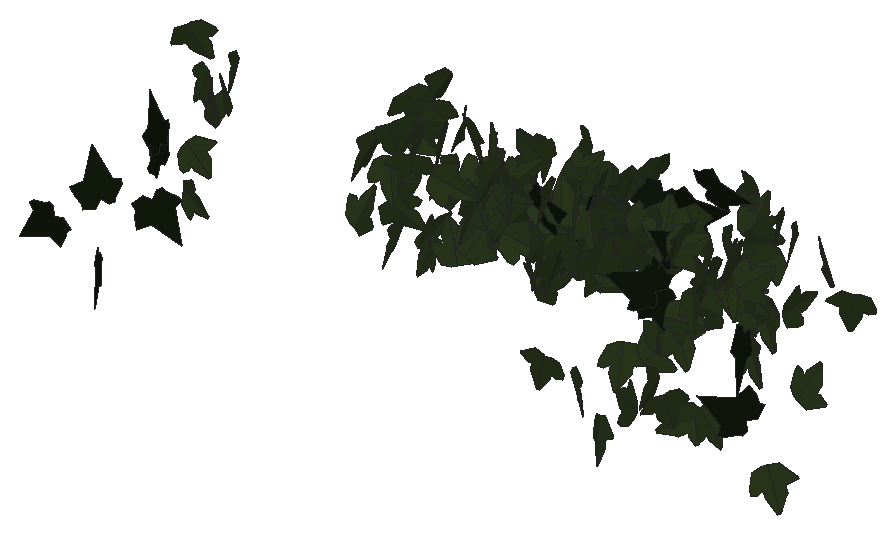
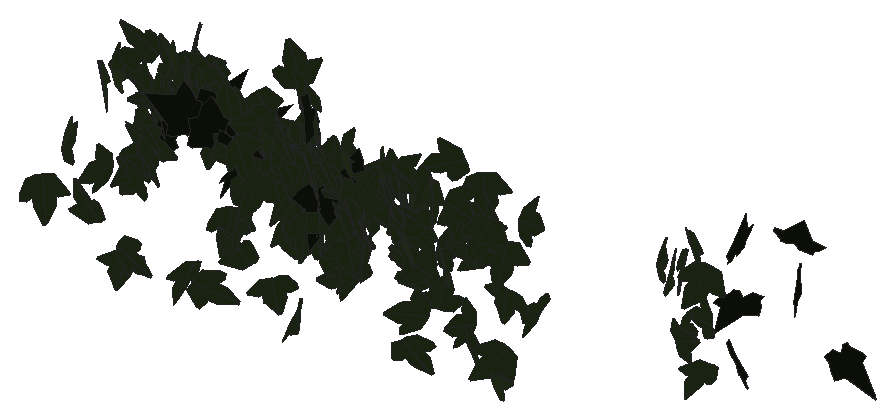
# SketchUp Ruby script. Lengths in inches.
U = 1.inch
M = Sketchup.active_model
def pt(a) = Geom::Point3d.new(a.map { |v| v * U })
def face(e, loops, mat)
  f = e.add_face(loops[0].map { |a| pt(a) })
  loops[1..].each { |l| e.add_face(l.map { |a| pt(a) }).erase! }
  f.material = f.back_material = mat if mat
  f
end
# faces: each face lists its corners as indices into pts; further lists are holes
def faces(e, pts, list, mat = nil) = list.each { |f| face(e, (f[0].is_a?(Array) ? f : [f]).map { |l| l.map { |i| pts[i] } }, mat) }
# xy, xz, yz: faces in a plane at the given z, y or x. An outline is a flat list of corners, or four numbers for a rectangle; further outlines are holes
def ring(l) = l.size == 4 ? [[l[0], l[1]], [l[2], l[1]], [l[2], l[3]], [l[0], l[3]]] : l.each_slice(2).to_a
def flat(e, list, mat, &to3) = list.each { |f| face(e, (f[0].is_a?(Array) ? f : [f]).map { |l| ring(l).map { |u, v| to3.(u, v) } }, mat) }
def xy(e, z, list, mat = nil) = flat(e, list, mat) { |x, y| [x, y, z] }
def xz(e, y, list, mat = nil) = flat(e, list, mat) { |x, z| [x, y, z] }
def yz(e, x, list, mat = nil) = flat(e, list, mat) { |y, z| [x, y, z] }
def lines(e, pts, list) = list.each { |a, b| e.add_line(pt(pts[a]), pt(pts[b])) }
# prism: a flat outline (further loops are holes) pulled along v
def prism(e, loops, v, mat = nil)
  f = face(e, loops, mat); d = Geom::Vector3d.new(v.map { |x| x * U })
  f.pushpull(f.normal.samedirection?(d) ? d.length : -d.length)
end
def box(e, o, s, mat = nil) = prism(e, [[o, [o[0] + s[0], o[1], o[2]], [o[0] + s[0], o[1] + s[1], o[2]], [o[0], o[1] + s[1], o[2]]]], [0, 0, s[2]], mat)
def at(x, y, z, deg = 0) = Geom::Transformation.translation(pt([x, y, z])) * Geom::Transformation.rotation(ORIGIN, Z_AXIS, deg.degrees)
def axes(o, x, y, z) = Geom::Transformation.new([*x, 0, *y, 0, *z, 0, *pt(o).to_a, 1])
def part(name) = M.definitions.add(name)
# library, detail: a bought-in or finely detailed component or shape, given as its bounding box
def library(name, o, s) = part(name).tap { |d| box(d.entities, o, s) }
def detail(e, o, s) = box(e.add_group.entities, o, s)
def put(e, d, t, mat = nil) = e.add_instance(d, t).tap { |i| i.material = mat if mat }
def group(e, t, mat = nil) = e.add_group.tap { |g| g.transformation = t; g.material = mat if mat }.entities
root = M.entities
M.materials.add("efeu1").color = [18, 25, 13]
M.materials.add("efeu2").color = [43, 57, 29]
c1 = part("ivyleaf_9")
p = [[1.54,2.16,1.25],[1.36,2.04,1.19],[-0.21,0.99,0.68],[-0.71,1.11,0.82],[-0.85,0.86,0.67],[-0.8,0.17,0.21],
  [-0.9,-0.01,0.1],[-0.67,-0.16,-0.02],[-0.08,-0.08,-0.05],[-0.03,-0.6,-0.4],[0.65,-0.88,-0.66],[0.83,-0.6,-0.49],
  [1.29,-0.42,-0.43],[1.8125,-0.07,-0.26],[1.21,0.44,0.15]]
faces(c1.entities,p,[[0,1,2,3,4,5,6,7,8,9,10,11,12,13,14]],"efeu1")
c2 = part("ivyleaf_10")
p = [[0,0.5,-0.03],[-0.0625,2.02,-0.43],[-0.19,2.01,-0.46],[-0.54,1.05,-0.29],[-0.52,0.625,-0.18],[-0.83,0.76,-0.28],
  [-1.16,0.64,-0.33],[-1.15,0.33,-0.24],[-0.77,-0.39,0.02],[-0.3,-0.51,0.16],[0.04,-0.48,0.23],[-0.02,2.01,-0.4375],
  [-0.06,2.01,-0.43],[0.04,-0.49,0.23],[0.67,-0.49,0.14],[1.38,0.36,-0.2],[1.375,0.51,-0.24],[0.81,0.65,-0.19],
  [0.62,0.59,-0.15],[0.6,1.09,-0.28],[0.5,1.23,-0.31]]
faces(c2.entities,p,[[0,1,2,3,4,5,6,7,8,9,10],[11,12,0,13,14,15,16,17,18,19,20]],"efeu2")
put(root,c1,axes([6.62,220.39,191.89],[0.08474,0.05698,-0.44102],[-0.36341,-0.25807,-0.10081],[-0.28542,0.34551,-0.00257]))
put(root,c1,axes([7.72,223.3,192.57],[-0.0591,0.13715,0.42554],[-0.18368,0.37221,-0.15341],[-0.42835,-0.17853,0.00707]))
put(root,c2,axes([7.66,224.63,195.72],[-0.39862,-0.20713,-0.21955],[0.18919,0.11193,-0.44909],[0.23519,-0.4411,-0.01086]))
put(root,c2,axes([8.375,224.53,193.77],[-0.12811,0.13937,-0.41041],[-0.29675,0.28346,0.19001],[0.34094,0.29909,0.01116]))
put(root,c2,axes([8.41,224.7,193.5625],[0.22777,-0.02241,0.39499],[-0.40902,0.02905,0.2205],[-0.03919,-0.43345,-0.00564]))
put(root,c2,axes([8.05,224.16,192.64],[0.17645,0.33449,0.23405],[0.08873,0.2101,-0.38681],[-0.42627,0.1822,0.01636]))
put(root,c1,axes([9.04,219.28,193.8],[-0.46437,-0.04223,0.05269],[0.05481,0.00155,0.44931],[-0.0455,0.43294,0.00353]))
put(root,c1,axes([9.17,221.48,194.49],[-0.06039,-0.34783,0.26538],[0.11564,0.23807,0.36189],[-0.45132,0.10754,0.05722]))
put(root,c2,axes([9.23,223.2,195.57],[0.34503,-0.25966,-0.14612],[-0.10667,0.10109,-0.42786],[0.30048,0.33404,0.01589]))
put(root,c2,axes([9.32,223.37,195.05],[-0.29865,0.28351,0.18715],[-0.13729,0.12738,-0.41187],[-0.33567,-0.30434,0.00195]))
put(root,c2,axes([9.35,223.99,194.58],[-0.30468,0.32137,0.08294],[0.05183,-0.06398,0.44469],[0.35383,0.2861,0.00628]))
put(root,c2,axes([9.25,224.39,195.38],[0.05361,-0.11993,0.43179],[0.28423,-0.3231,-0.12979],[0.37021,0.26542,0.03711]))
put(root,c1,axes([9.28,221.13,192.92],[-0.01956,-0.2665,-0.35706],[0.0522,0.34026,-0.27733],[0.46648,-0.04925,0.01606]))
put(root,c1,axes([9.35,218.83,192.27],[-0.04609,0.0276,-0.4493],[0.41825,-0.19156,-0.05252],[-0.20893,-0.38957,-0.00601]))
put(root,c2,axes([9.45,222.25,192.67],[0.05716,-0.02684,0.44817],[0.46238,-0.05297,-0.05811],[0.0604,0.43093,0.02077]))
put(root,c2,axes([13.3,224.23,192.48],[0.10905,0.23457,-0.42788],[0.04645,0.43145,0.24837],[0.48575,-0.09392,0.07231]))
put(root,c2,axes([13.16,225.92,192.0625],[-0.33539,-0.14457,-0.34149],[0.31242,0.13788,-0.36522],[0.19977,-0.45835,-0.00216]))
put(root,c2,axes([13.29,225.86,191.4],[0.13832,-0.26853,0.39845],[0.1786,-0.35619,-0.30204],[0.44606,0.22588,-0.00262]))
put(root,c2,axes([13.51,225.32,194.64],[-0.28836,-0.39178,-0.11559],[0.07938,0.08504,-0.48628],[0.40068,-0.2988,0.01315]))
put(root,c2,axes([13.34,225.4,193.48],[0.47228,0.06519,0.15068],[0.14937,0.01982,-0.47675],[-0.06813,0.49534,-0.00076]))
put(root,c2,axes([13.72,225.78,195.45],[-0.28246,-0.33605,-0.23935],[0.16991,0.16958,-0.4386],[0.37596,-0.32911,0.0184]))
put(root,c2,axes([13.81,224.09,194.83],[0.07673,-0.26627,0.41619],[0.14901,-0.38909,-0.27641],[0.47107,0.16645,0.01965]))
put(root,c2,axes([14.08,225.53,194.98],[-0.08698,-0.46505,0.16174],[-0.02901,-0.15912,-0.47312],[0.49152,-0.09169,0.00069]))
put(root,c2,axes([13.97,225.67,194.46],[0.30077,0.01806,-0.39901],[0.34839,0.23244,0.27313],[0.19535,-0.44232,0.12724]))
put(root,c2,axes([14.29,225.54,194.77],[0.15304,-0.4027,0.25379],[0.11799,-0.22617,-0.43003],[0.46115,0.19151,0.0258]))
put(root,c2,axes([14.45,226.22,196],[0.05074,-0.34663,0.35675],[0.03482,-0.35525,-0.35012],[0.4962,0.06037,-0.01191]))
put(root,c2,axes([14.61,225.64,195.53],[-0.44168,-0.23434,0.00203],[-0.00168,-0.00117,-0.5],[0.23434,-0.44168,0.00025]))
put(root,c2,axes([14.41,225.49,195.16],[0.15056,-0.085,-0.46916],[0.40127,-0.24314,0.17282],[-0.25752,-0.42855,-0.005]))
put(root,c2,axes([14.8,225.17,192],[0.03964,-0.18016,0.46473],[-0.12442,0.44786,0.18424],[-0.48265,-0.13025,-0.00933]))
put(root,c2,axes([14.85,225.1875,191.83],[0.40949,-0.26393,-0.11251],[-0.09576,0.05911,-0.48717],[0.27046,0.42053,-0.00214]))
put(root,c2,axes([15.03,225.49,194.99],[0.23648,-0.25557,0.35884],[0.23263,-0.27341,-0.34803],[0.37412,0.33156,-0.0104]))
put(root,c2,axes([15.41,226.78,191.91],[0.41003,0.12376,-0.25799],[-0.24692,-0.07477,-0.4283],[-0.14459,0.47864,-0.00019]))
put(root,c2,axes([15.52,223.65,195.15],[-0.41514,-0.27022,0.06813],[-0.05692,-0.03745,-0.49534],[0.2728,-0.41902,0.00033]))
put(root,c2,axes([15.36,225.42,194.09],[0.04545,-0.15081,0.47454],[0.15025,-0.45015,-0.15744],[0.47472,0.15691,0.0044]))
put(root,c2,axes([15.38,225.32,193.37],[0.37608,-0.32507,0.05377],[-0.03541,0.04125,0.49704],[-0.32758,-0.37766,0.00801]))
put(root,c2,axes([15.22,223.69,194.46],[0.11743,-0.18963,-0.44749],[0.3391,-0.29783,0.21519],[-0.34816,-0.35404,0.05866]))
put(root,c2,axes([15.79,225.3,195.6],[0.1172,-0.38501,-0.2967],[-0.07918,0.28601,-0.40241],[0.47958,0.14131,0.00607]))
put(root,c2,axes([15.9375,226.14,193.88],[0.27919,-0.32382,0.25922],[-0.16116,0.20323,0.42746],[-0.3822,-0.32224,0.0091]))
put(root,c2,axes([15.95,224.86,192.09],[0.39413,0.29679,0.08111],[-0.06919,-0.04294,0.49332],[0.29979,-0.40009,0.00722]))
put(root,c2,axes([16.01,225.62,192.08],[-0.03452,-0.16414,0.47103],[0.08097,0.46405,0.16764],[-0.49219,0.08785,-0.00545]))
put(root,c2,axes([16.09,225.25,195.68],[-0.39567,0.28255,-0.11667],[0.09466,-0.0682,-0.4862],[-0.29067,-0.40683,0.00048]))
put(root,c2,axes([16.18,225.33,193.1875],[-0.13932,-0.34499,0.33402],[0.16556,0.29197,0.3706],[-0.45076,0.21386,0.03288]))
put(root,c2,axes([16.375,225.1,194.29],[0.32425,0.14629,-0.35137],[0.27946,0.22185,0.35026],[0.25838,-0.42354,0.0621]))
put(root,c2,axes([16.49,224.77,192.52],[0.42198,0.07793,-0.25663],[0.25187,0.04923,0.42911],[0.09215,-0.49143,0.00229]))
put(root,c2,axes([16.71,224.7,193.77],[0.00475,0.31989,-0.38425],[-0.05019,-0.38202,-0.31866],[-0.49745,0.0416,0.02848]))
put(root,c2,axes([16.74,225.23,193.6],[0.11918,-0.43362,0.21855],[-0.05328,0.212,0.44968],[-0.48266,-0.13048,0.00433]))
put(root,c2,axes([16.94,225.08,194.97],[0.34988,-0.19717,0.29783],[-0.25883,0.14734,0.40162],[-0.24614,-0.43522,0.00103]))
put(root,c2,axes([17.02,225.06,195.1],[0.14865,-0.29227,-0.37747],[-0.17175,0.33613,-0.3279],[0.44543,0.22714,-0.00047]))
put(root,c2,axes([16.7,223.27,195.2],[0.14093,0.09653,0.46992],[0.38928,0.26322,-0.17081],[-0.28036,0.414,-0.00096]))
put(root,c2,axes([16.84,224.76,194.02],[-0.26911,-0.02808,0.42046],[0.37068,-0.25307,0.22035],[0.20044,0.43031,0.15703]))
put(root,c2,axes([16.9,225.05,193.75],[0.29915,-0.19917,0.34762],[0.28548,-0.1984,-0.35936],[0.28109,0.41348,-0.00498]))
put(root,c2,axes([17.57,226.41,194.9],[0.27556,-0.24539,-0.33742],[-0.25498,0.22103,-0.36896],[0.33024,0.37541,-0.00333]))
put(root,c2,axes([17.42,224.58,195.1875],[0.0096,-0.3895,0.31336],[0.04761,-0.31128,-0.38838],[0.49764,0.0373,0.03111]))
put(root,c2,axes([17.6,226.1,194.97],[-0.33472,-0.25347,-0.2715],[-0.22033,-0.15874,0.41983],[-0.29903,0.40069,-0.00543]))
put(root,c2,axes([17.21,224.73,193.71],[0.29997,-0.131,-0.37797],[0.37101,-0.08552,0.32409],[-0.14956,-0.4749,0.0459]))
put(root,c2,axes([17.33,226.1,194.3],[0.2026,-0.16963,0.42447],[0.34792,-0.24392,-0.26354],[0.29648,0.40216,0.0192]))
put(root,c2,axes([17.55,225.0625,195.03],[0.3624,-0.33389,0.08473],[0.06444,-0.0551,-0.49276],[0.3384,0.36807,0.0031]))
put(root,c2,axes([17.55,226.03,194.52],[0.25137,-0.22348,0.36996],[0.28531,-0.23569,-0.33623],[0.32467,0.38014,0.00903]))
put(root,c2,axes([18.04,224.83,194.08],[-0.07096,-0.33562,0.36376],[-0.07113,-0.35675,-0.34303],[0.4898,-0.10043,0.00289]))
put(root,c2,axes([17.85,224.68,194.9],[0.09707,0.1489,-0.46734],[0.25252,0.39324,0.17774],[0.42049,-0.27054,0.00114]))
put(root,c2,axes([17.95,225.04,194.44],[-0.36224,-0.16989,-0.29986],[0.2833,0.10097,-0.39943],[0.19627,-0.45928,0.02311]))
put(root,c2,axes([17.72,224.44,194.87],[0.00355,-0.05365,0.4971],[0.49174,0.09029,0.00623],[-0.09044,0.48884,0.05341]))
put(root,c2,axes([18.17,225.74,193.35],[0.34083,0.35619,-0.08346],[-0.05871,-0.05934,-0.49298],[-0.36109,0.34585,0.00138]))
put(root,c2,axes([18.55,225.63,193.89],[-0.3328,-0.13952,0.34609],[-0.3194,-0.13326,-0.36087],[0.19293,-0.46128,-0.00043]))
put(root,c2,axes([18.25,225.08,194.3],[-0.43076,-0.22696,-0.11374],[0.10026,0.05372,-0.48689],[0.23323,-0.44227,-0.00077]))
put(root,c2,axes([18.1,224.38,195.05],[0.33768,-0.27701,0.24338],[0.19895,-0.14099,-0.43651],[0.31046,0.39165,0.01501]))
put(root,c2,axes([18.49,224.79,192.22],[-0.37,0.33315,-0.04593],[-0.03519,0.02956,0.49788],[0.33445,0.37167,0.00157]))
put(root,c2,axes([18.41,225.67,194.11],[0.46843,-0.1729,-0.02612],[-0.02217,0.01535,-0.49927],[0.17345,0.4689,0.00672]))
put(root,c2,axes([18.48,225.12,192.61],[-0.01607,-0.3016,-0.39847],[0.03915,0.39669,-0.30183],[0.49821,-0.04091,0.01087]))
put(root,c2,axes([18.36,224.09,193.76],[0.15388,0.1628,0.44701],[0.31284,0.31931,-0.22399],[-0.3584,0.34862,-0.00359]))
put(root,c2,axes([18.63,225.07,192.1],[0.03132,0.03793,-0.49757],[0.24568,0.43277,0.04846],[0.43435,-0.24752,0.00847]))
put(root,c2,axes([18.57,225.06,194],[0.35286,0.08922,-0.34282],[0.27287,0.24011,0.34335],[0.22589,-0.42941,0.12076]))
put(root,c2,axes([19.03,226.25,195.67],[0.19183,-0.25033,-0.38799],[-0.23948,0.30528,-0.31536],[0.39478,0.30682,-0.00277]))
put(root,c2,axes([18.91,225.51,192.81],[-0.03119,-0.33564,0.36929],[-0.01828,-0.36899,-0.33691],[0.49869,-0.03452,0.01074]))
put(root,c2,axes([19.1,225.86,193.8],[0.17138,-0.21626,-0.41697],[-0.21891,0.35593,-0.27458],[0.41558,0.27667,0.02732]))
put(root,c2,axes([18.93,226.46,194.04],[-0.18334,-0.45031,-0.11667],[0.05898,0.10189,-0.48594],[0.46142,-0.19194,0.01576]))
put(root,c1,axes([19,225.6,194.4],[0.17348,0.46636,0.04909],[0.01626,0.04633,-0.49758],[-0.46866,0.17424,0.00091]))
put(root,c1,axes([18.85,224.66,194.45],[0.04825,-0.05771,0.49431],[0.31398,-0.38179,-0.07521],[0.38612,0.31766,-0.0006]))
put(root,c2,axes([19.04,224.3,193.69],[-0.14274,0.04928,0.47665],[0.29632,-0.38178,0.12821],[0.37659,0.31909,0.07979]))
put(root,c2,axes([19.13,224.62,195.23],[0.1947,-0.33182,0.31936],[0.16078,-0.27593,-0.38472],[0.43156,0.2525,-0.00075]))
put(root,c2,axes([18.99,225.54,194.85],[0.33287,-0.1466,-0.34308],[0.30612,-0.15553,0.36346],[-0.21329,-0.45202,-0.01379]))
put(root,c2,axes([19.24,225.5,194.72],[0.06339,-0.14926,0.47297],[0.15745,-0.4461,-0.16188],[0.47031,0.16946,-0.00956]))
put(root,c2,axes([19.07,225.875,195.03],[0.38197,-0.06183,-0.31667],[0.31728,-0.01718,0.38606],[-0.05862,-0.49587,0.02611]))
put(root,c2,axes([19.57,225.3,194.87],[0.20005,-0.41291,-0.1987],[-0.08177,0.18117,-0.45879],[0.45088,0.21606,0.00496]))
put(root,c2,axes([19.5625,224.87,193.85],[-0.25182,-0.42019,-0.10014],[0.06085,0.08025,-0.48975],[0.42765,-0.25884,0.01072]))
put(root,c2,axes([19.53,226.32,193.76],[0.06059,-0.25793,0.42403],[0.12001,-0.40689,-0.26465],[0.48159,0.13384,0.0126]))
put(root,c2,axes([19.58,224.57,194.65],[0.46506,0.18104,0.03079],[-0.0357,0.0069,0.49868],[0.18013,-0.46602,0.01934]))
put(root,c2,axes([19.66,224.14,193.57],[0.02094,-0.49681,0.05237],[0.00548,-0.05218,-0.49724],[0.49953,0.0214,0.00326]))
put(root,c2,axes([19.26,225.57,193.02],[0.08194,-0.04268,0.49139],[0.49324,0.0057,-0.08175],[0.00137,0.49814,0.04304]))
put(root,c2,axes([19.82,225.875,195.21],[-0.11686,-0.39232,0.28711],[-0.03136,-0.28859,-0.4071],[0.48514,-0.11315,0.04285]))
put(root,c2,axes([19.75,224.9,194.43],[-0.41027,-0.26654,-0.10312],[0.08449,0.05923,-0.48924],[0.27302,-0.41887,-0.00356]))
put(root,c2,axes([19.59,225.9,194.98],[0.4247,0.22091,0.14432],[0.12777,0.0671,-0.47872],[-0.23087,0.44351,0.00054]))
put(root,c2,axes([19.68,224.93,193.16],[0.44619,-0.08024,-0.21088],[0.21126,-0.01559,0.45291],[-0.07926,-0.49327,0.01999]))
put(root,c2,axes([19.72,225.17,195.01],[-0.31906,-0.04005,-0.38288],[0.3779,0.06227,-0.32143],[0.07343,-0.49449,-0.00946]))
put(root,c2,axes([20.12,224.71,193.82],[-0.33527,-0.36707,0.05345],[-0.03581,-0.03968,-0.49713],[0.3692,-0.33718,0.00032]))
put(root,c2,axes([19.9,225.41,192.57],[-0.37103,-0.14722,0.3011],[0.28169,0.10643,0.39915],[-0.18162,0.46583,0.00397]))
put(root,c2,axes([19.95,224.73,195.37],[0.30659,-0.22934,0.32157],[0.2516,-0.2004,-0.38281],[0.30447,0.39654,-0.00748]))
put(root,c2,axes([20.38,222.85,191.5],[-0.4674,-0.0774,0.15984],[-0.15567,-0.03808,-0.47362],[0.08549,-0.4925,0.0115]))
put(root,c2,axes([20.24,225.37,195.55],[0.21383,-0.43824,0.11055],[0.04336,-0.10184,-0.48759],[0.44989,0.21811,-0.00555]))
put(root,c2,axes([20.2,226.76,194.85],[-0.20374,-0.36744,-0.27107],[0.15863,0.22138,-0.41932],[0.42817,-0.25686,0.02637]))
put(root,c2,axes([20.21,225.65,195.57],[0.45902,-0.19679,0.02394],[0.02201,-0.00944,-0.49943],[0.19702,0.45955,0]))
put(root,c2,axes([20.37,225.36,194.03],[-0.07269,-0.35235,-0.34723],[0.08633,0.33654,-0.35957],[0.4871,-0.11222,0.01191]))
put(root,c2,axes([20.49,224.96,193.14],[-0.17261,-0.33654,-0.32703],[0.18286,0.27267,-0.37711],[0.43217,-0.24979,0.02895]))
put(root,c1,axes([20.93,223.78,195.38],[-0.18517,0.1319,-0.44533],[-0.38706,0.22115,0.22644],[0.2567,0.4286,0.0202]))
put(root,c2,axes([20.43,225.03,194.93],[-0.19149,-0.01202,0.46172],[0.46182,0.00279,0.19161],[-0.00719,0.49985,0.01004]))
put(root,c2,axes([20.88,226.72,195.625],[-0.05915,-0.48856,0.08836],[-0.01415,-0.08729,-0.49212],[0.49629,-0.06072,-0.0035]))
put(root,c2,axes([20.82,225.73,195.61],[0.12954,-0.29289,0.38397],[0.16402,-0.34723,-0.3202],[0.45422,0.20891,0.00612]))
put(root,c2,axes([20.58,225.45,195],[0.02859,-0.07527,0.49347],[0.49893,-0.01133,-0.03064],[0.01579,0.49417,0.07446]))
put(root,c2,axes([20.8,224.61,193.44],[-0.21241,-0.18387,0.41361],[0.29807,0.28702,0.28067],[-0.34064,0.3658,-0.01232]))
put(root,c2,axes([21.05,223.83,194.95],[-0.05244,-0.34585,-0.35726],[0.0763,0.34939,-0.34944],[0.49135,-0.09117,0.01614]))
put(root,c2,axes([21.03,225.14,190.97],[0.35236,0.34923,-0.06231],[-0.04829,-0.03978,-0.49607],[-0.35144,0.35561,0.00569]))
put(root,c2,axes([21.29,225.2,194.76],[-0.12682,-0.42843,-0.22441],[0.05649,0.21729,-0.44676],[0.48034,-0.13867,-0.00671]))
put(root,c2,axes([21.27,223.97,189.49],[-0.08001,0.41756,-0.26314],[0.05146,-0.25807,-0.42515],[-0.49087,-0.09512,-0.00168]))
put(root,c2,axes([21.38,223.43,194.96],[0.39684,-0.30409,0.0068],[0.00565,-0.00382,-0.49995],[0.30411,0.39688,0.0004]))
put(root,c2,axes([21.67,225.625,193.65],[-0.03376,0.04335,0.49697],[-0.29032,-0.40678,0.01576],[0.40568,-0.28749,0.05264]))
put(root,c2,axes([21.13,223.83,194.34],[-0.22979,-0.06859,0.43874],[0.43488,0.06525,0.23796],[-0.0899,0.49096,0.02966]))
put(root,c2,axes([21.46,225.28,194.85],[0.00458,0.0267,-0.49927],[-0.00972,-0.49919,-0.02679],[-0.49988,0.00995,-0.00405]))
put(root,c1,axes([21.59,226.02,195.29],[-0.42292,-0.16701,-0.20795],[0.19477,0.07294,-0.45469],[0.18221,-0.46561,0.00336]))
put(root,c2,axes([21.38,223.36,195.66],[0.40843,-0.07369,0.27885],[0.27393,-0.05222,-0.41501],[0.09029,0.49177,-0.00228]))
put(root,c2,axes([21.75,224.76,194.56],[-0.23211,-0.44277,0.00882],[-0.003,-0.00839,-0.49992],[0.44285,-0.23212,0.00124]))
put(root,c2,axes([21.71,222.43,191.61],[-0.18716,0.21762,-0.40941],[0.24258,-0.3303,-0.28646],[-0.39513,-0.30585,0.01806]))
put(root,c2,axes([21.89,224.67,195.07],[0.06038,0.14774,-0.47384],[0.19993,0.42966,0.15944],[0.45429,-0.20872,-0.00719]))
put(root,c2,axes([22.26,224.93,191.82],[-0.03629,0.36861,-0.33587],[-0.05377,0.3319,0.37006],[0.49577,0.06298,0.01555]))
put(root,c2,axes([22.6,223.73,195.05],[-0.38571,-0.09087,0.30491],[-0.29826,-0.06353,-0.39624],[0.11076,-0.48755,-0.00519]))
put(root,c2,axes([22.07,225.01,191.31],[0.37235,0.03762,-0.33157],[0.33045,0.02762,0.37422],[0.04647,-0.49782,-0.00429]))
put(root,c2,axes([22.64,224.53,195.5],[0.30532,-0.32205,-0.23035],[-0.16252,0.16332,-0.44375],[0.36106,0.34585,-0.00495]))
put(root,c2,axes([22.49,222.35,195.18],[-0.26332,-0.41948,0.06855],[0.03857,0.05672,0.49527],[-0.42329,0.26612,0.00249]))
put(root,c2,axes([22.44,224.43,194.03],[-0.00645,-0.01194,-0.49982],[0.31747,0.38605,-0.01332],[0.38622,-0.31753,0.0026]))
put(root,c2,axes([22.72,224.75,195.12],[0.35175,0.34112,-0.09956],[0.06788,0.07301,0.48996],[0.34881,-0.3582,0.00505]))
put(root,c1,axes([23.05,223.87,194],[-0.0308,-0.00895,0.49897],[-0.46412,-0.18324,-0.03194],[0.18343,-0.46513,0.00298]))
put(root,c1,axes([22.65,224.39,193.59],[0.17723,-0.42512,-0.19458],[-0.07011,0.18158,-0.46056],[0.46225,0.19053,0.00476]))
put(root,c2,axes([23.13,227.74,195.11],[0.17668,-0.16573,-0.4374],[-0.33275,0.28407,-0.24204],[0.32873,0.37661,-0.00992]))
put(root,c1,axes([22.47,225.86,195.15],[0.11136,-0.04221,0.48561],[0.44558,-0.19314,-0.11896],[0.19762,0.45926,-0.0054]))
put(root,c2,axes([23.45,224.97,190.02],[0.22394,0.09604,-0.43661],[-0.41721,-0.13051,-0.2427],[-0.16058,0.47301,0.02168]))
put(root,c1,axes([22.8,226.43,195.69],[0.20874,-0.10072,0.44304],[0.38247,-0.22421,-0.23118],[0.24524,0.43541,-0.01655]))
put(root,c1,axes([23.35,224.75,194.81],[0.09694,0.0658,0.48608],[-0.39686,-0.28068,0.11715],[0.28828,-0.40852,-0.00219]))
put(root,c2,axes([23.23,223.65,191.5],[0.02,-0.05431,0.49664],[0.26618,-0.41946,-0.05659],[0.42278,0.26666,0.01213]))
put(root,c2,axes([23.35,227.4375,194.33],[0.14145,0.34543,-0.33267],[0.11609,0.31186,0.37318],[0.46531,-0.18281,0.00802]))
put(root,c2,axes([23.82,227.58,192.01],[0.16765,-0.07177,-0.46556],[-0.42555,0.18882,-0.18235],[0.20199,0.45738,0.00222]))
put(root,c2,axes([23.15,224.57,195.13],[0.16387,-0.01961,-0.47198],[0.47057,-0.03695,0.16492],[-0.04135,-0.49825,0.00635]))
put(root,c2,axes([23.67,224.1,195.66],[0.17681,-0.46078,-0.08015],[-0.02569,0.07599,-0.49352],[0.46699,0.17864,0.0032]))
put(root,c2,axes([23.71,223.55,191.25],[-0.29269,-0.3895,-0.11235],[0.06875,0.08887,-0.48721],[0.39951,-0.30065,0.00153]))
put(root,c2,axes([23.79,224.4,195.78],[0.05729,-0.48231,0.11873],[0.01024,-0.11834,-0.48569],[0.4966,0.05808,-0.00368]))
put(root,c2,axes([23.8,227.05,194.49],[-0.15048,-0.24854,-0.40692],[0.18463,0.36304,-0.29002],[0.43962,-0.23754,-0.01749]))
put(root,c2,axes([23.61,224.58,196],[0.39877,0.08548,0.28926],[0.28339,0.05802,-0.40783],[-0.10329,0.48921,-0.00218]))
put(root,c2,axes([23.9375,224.89,190.27],[0.01667,0.46732,0.17702],[0.00872,0.17682,-0.46761],[-0.49965,0.01868,-0.00225]))
put(root,c2,axes([23.68,224.08,195.3],[0.28125,-0.03055,-0.41227],[0.4131,0.00191,0.28168],[-0.01564,-0.49906,0.02632]))
put(root,c2,axes([24.07,221.6875,191.94],[-0.18011,0.3785,0.27258],[0.11278,-0.24819,0.41914],[0.45259,0.21247,0.00403]))
put(root,c2,axes([24.17,223.44,193.36],[0.18904,0.45,0.10847],[0.04282,0.09967,-0.48809],[-0.4609,0.19382,-0.00086]))
put(root,c2,axes([24.28,224.74,194.52],[-0.05411,-0.1106,-0.4846],[-0.06655,-0.48146,0.11731],[-0.49259,0.0772,0.03739]))
put(root,c2,axes([24.52,224.25,195.375],[0.23675,-0.37673,-0.22808],[-0.12427,0.19128,-0.44494],[0.4225,0.26737,-0.00307]))
put(root,c2,axes([24.16,223.36,193.84],[-0.05056,-0.03514,-0.49619],[0.49416,0.05358,-0.05414],[0.05698,-0.49588,0.02932]))
put(root,c2,axes([24.6875,224.77,195.51],[-0.26716,0.3405,0.25038],[-0.15716,0.19493,-0.43279],[-0.39234,-0.30994,0.00287]))
put(root,c2,axes([25.125,225.07,193.57],[0.04148,-0.02895,-0.49743],[-0.47118,0.16008,-0.04861],[0.16207,0.4728,-0.014]))
put(root,c2,axes([24.89,224.8,195.18],[0.04019,-0.3925,-0.30712],[-0.04025,0.30456,-0.39449],[0.49675,0.05643,-0.00712]))
put(root,c2,axes([24.83,225.98,193.05],[0.37212,-0.02327,0.33314],[0.33249,-0.02093,-0.37285],[0.0313,0.49902,-0.00011]))
put(root,c2,axes([24.95,223,194.83],[0.38147,-0.16306,0.2791],[0.25684,-0.10923,-0.41485],[0.19626,0.45987,0.00042]))
put(root,c2,axes([25.6,223.15,194.61],[-0.00582,0.01432,0.49976],[-0.49141,-0.09221,-0.00308],[0.09207,-0.49122,0.01514]))
put(root,c2,axes([24.92,225.22,193.56],[0.08351,-0.04101,-0.49127],[0.43586,-0.22666,0.09301],[-0.23033,-0.44378,-0.0021]))
put(root,c2,axes([24.93,225.31,195.26],[0.0258,-0.0059,0.4993],[0.48803,-0.10547,-0.02646],[0.10563,0.48871,0.00031]))
put(root,c2,axes([25.03,224.32,194.49],[0.01028,-0.06072,0.49619],[0.3162,0.38519,0.04059],[-0.38719,0.31295,0.04631]))
put(root,c2,axes([25.14,223.19,195.36],[-0.13981,0.06583,0.47552],[0.32545,-0.35108,0.14429],[0.35289,0.34987,0.05532]))
put(root,c2,axes([25.3,223.93,195.18],[0.19146,-0.45545,0.07686],[-0.02961,0.07093,0.49406],[-0.46094,-0.19374,0.00019]))
put(root,c2,axes([25.31,224.43,194.78],[0.49682,-0.02134,0.05209],[0.05232,0.00435,-0.49724],[0.02076,0.49953,0.00656]))
put(root,c2,axes([25.52,226.29,193.22],[0.03827,-0.06391,0.49442],[-0.10066,0.48467,0.07044],[-0.48827,-0.10493,0.02423]))
put(root,c2,axes([25.46,225.91,195.89],[0.16459,-0.18528,0.43426],[0.27688,-0.33463,-0.24771],[0.38243,0.32202,-0.00755]))
put(root,c2,axes([26.01,224.95,195.52],[0.27363,0.04087,-0.41648],[-0.41731,-0.01054,-0.27521],[-0.03127,0.49822,0.02834]))
put(root,c2,axes([25.97,225.85,195.66],[0.20999,-0.38612,-0.23835],[-0.11474,0.20892,-0.43953],[0.43902,0.23929,-0.00086]))
put(root,c2,axes([26.1,227.09,194.07],[-0.29295,0.29865,-0.27385],[-0.18818,0.199,0.41832],[0.35885,0.34815,-0.00419]))
put(root,c1,axes([26.04,223.75,193.75],[-0.31373,0.036,-0.38765],[0.38656,-0.03043,-0.31567],[-0.04632,-0.49777,-0.00874]))
put(root,c2,axes([26.31,227.81,193.14],[-0.43387,-0.23436,0.08267],[-0.07275,-0.03928,-0.49312],[0.23763,-0.43992,-0.00001]))
put(root,c2,axes([26.09,223.74,195.32],[0.29951,0.00557,-0.40033],[0.40026,0.00745,0.29956],[0.0093,-0.49991,0.00001]))
put(root,c2,axes([26.26,224.5,189.56],[0.36921,0.30258,0.14874],[0.11388,0.0957,-0.47736],[-0.31735,0.38637,0.00175]))
put(root,c2,axes([26.12,223.83,193.39],[0.3042,-0.07195,0.39024],[0.38345,-0.07324,-0.31241],[0.10212,0.48935,0.01062]))
put(root,c1,axes([26.75,222.87,192.0625],[0.0135,0.02463,0.49921],[-0.45933,-0.19629,0.02211],[0.19707,-0.4592,0.01733]))
put(root,c2,axes([26.33,225.77,191.4],[0.44231,-0.05268,-0.22713],[0.22542,-0.0278,0.44543],[-0.05956,-0.49644,-0.00084]))
